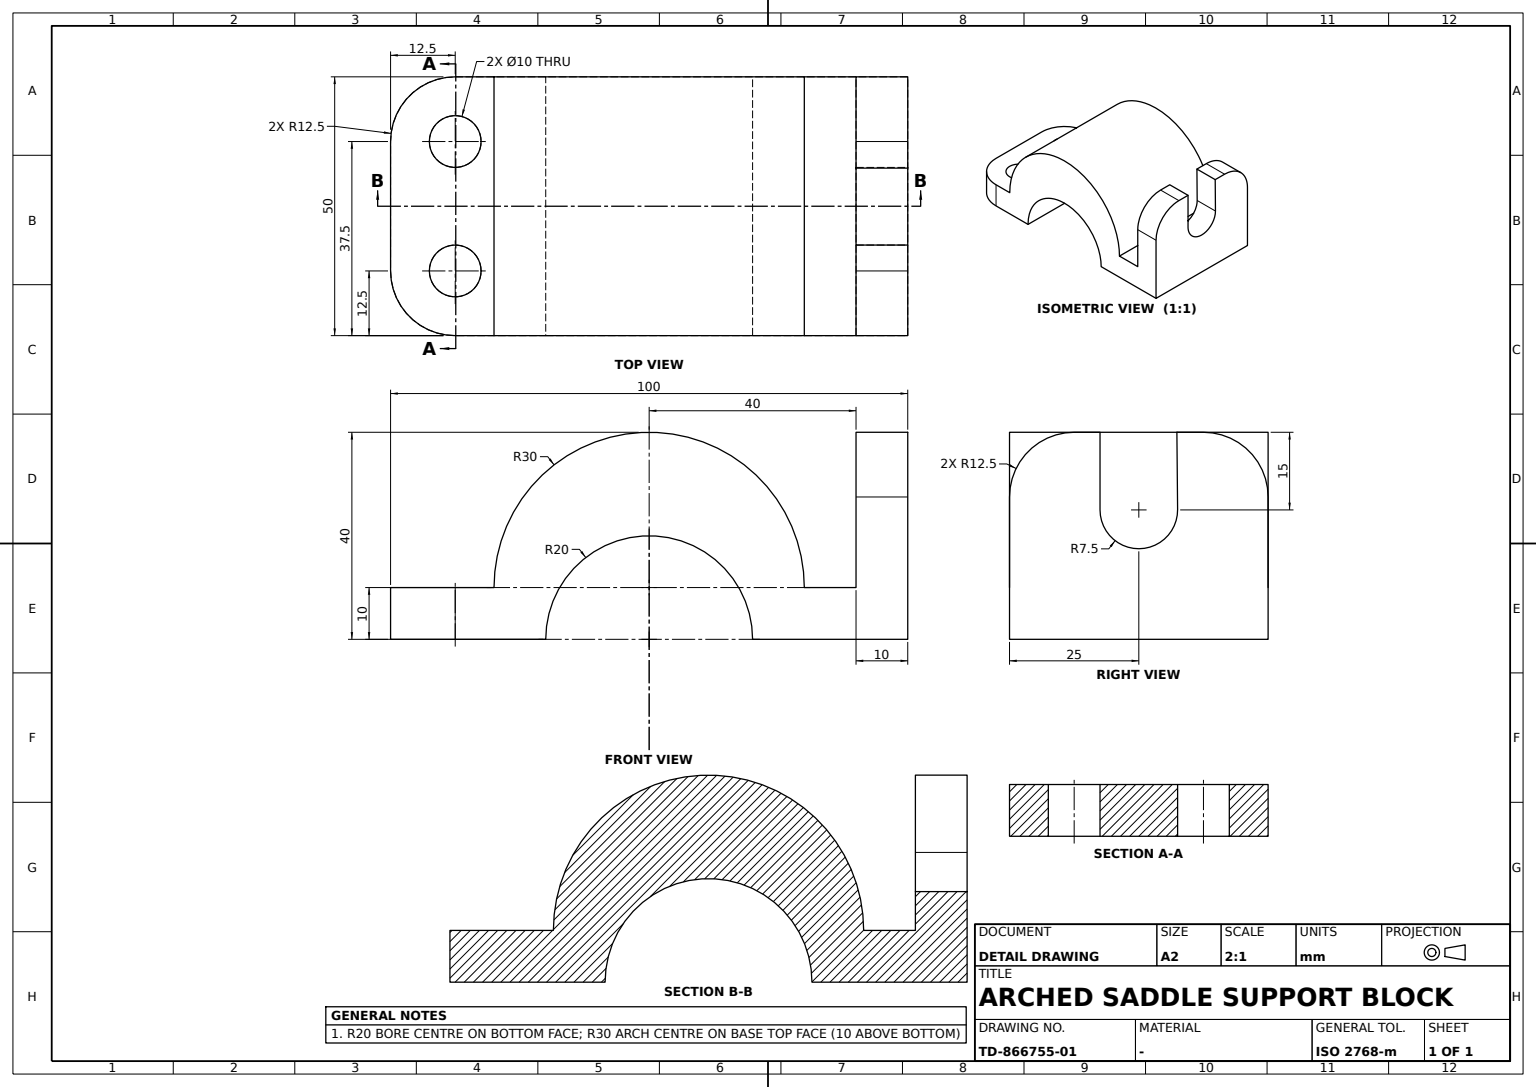
ISO-10303-21;
HEADER;
FILE_DESCRIPTION((''),'2;1');
FILE_NAME('','',(''),(''),'','','');
FILE_SCHEMA(('AUTOMOTIVE_DESIGN'));
ENDSEC;
DATA;
#1=APPLICATION_CONTEXT('');
#2=PRODUCT_CONTEXT('',#1,'mechanical');
#3=PRODUCT('','','',(#2));
#4=PRODUCT_DEFINITION_FORMATION('','',#3);
#5=PRODUCT_DEFINITION_CONTEXT('',#1,'design');
#6=PRODUCT_DEFINITION('','',#4,#5);
#7=PRODUCT_DEFINITION_SHAPE('','',#6);
#8=(LENGTH_UNIT()NAMED_UNIT(*)SI_UNIT(.MILLI.,.METRE.));
#9=(NAMED_UNIT(*)PLANE_ANGLE_UNIT()SI_UNIT($,.RADIAN.));
#10=(NAMED_UNIT(*)SI_UNIT($,.STERADIAN.)SOLID_ANGLE_UNIT());
#11=UNCERTAINTY_MEASURE_WITH_UNIT(LENGTH_MEASURE(0.005),#8,'distance_accuracy_value','');
#12=(GEOMETRIC_REPRESENTATION_CONTEXT(3)GLOBAL_UNCERTAINTY_ASSIGNED_CONTEXT((#11))GLOBAL_UNIT_ASSIGNED_CONTEXT((#8,#9,#10))REPRESENTATION_CONTEXT('',''));
#13=CARTESIAN_POINT('',(0.,-7.5,25.));
#14=VERTEX_POINT('',#13);
#15=CARTESIAN_POINT('',(-10.,-7.5,25.));
#16=VERTEX_POINT('',#15);
#17=CARTESIAN_POINT('',(-5.,-7.5,25.));
#18=DIRECTION('',(1.,0.,0.));
#19=VECTOR('',#18,1000.);
#20=LINE('',#17,#19);
#21=EDGE_CURVE('',#14,#16,#20,.F.);
#22=ORIENTED_EDGE('',*,*,#21,.T.);
#23=CARTESIAN_POINT('',(-10.,-7.5,40.));
#24=VERTEX_POINT('',#23);
#25=DIRECTION('',(0.,0.,1.));
#26=VECTOR('',#25,1000.);
#27=LINE('',#15,#26);
#28=EDGE_CURVE('',#16,#24,#27,.T.);
#29=ORIENTED_EDGE('',*,*,#28,.T.);
#30=CARTESIAN_POINT('',(0.,-7.5,40.));
#31=VERTEX_POINT('',#30);
#32=DIRECTION('',(-1.,0.,0.));
#33=VECTOR('',#32,1000.);
#34=LINE('',#30,#33);
#35=EDGE_CURVE('',#31,#24,#34,.T.);
#36=ORIENTED_EDGE('',*,*,#35,.F.);
#37=CARTESIAN_POINT('',(0.,-7.5,0.));
#38=LINE('',#37,#26);
#39=EDGE_CURVE('',#14,#31,#38,.T.);
#40=ORIENTED_EDGE('',*,*,#39,.F.);
#41=EDGE_LOOP('',(#22,#29,#36,#40));
#42=FACE_BOUND('',#41,.T.);
#43=DIRECTION('',(0.,-1.,0.));
#44=AXIS2_PLACEMENT_3D('',#13,#43,#25);
#45=PLANE('',#44);
#46=ADVANCED_FACE('',(#42),#45,.F.);
#47=CARTESIAN_POINT('',(-80.,-25.,10.));
#48=VERTEX_POINT('',#47);
#49=CARTESIAN_POINT('',(-20.,-25.,10.));
#50=VERTEX_POINT('',#49);
#51=CARTESIAN_POINT('',(-50.,-25.,10.));
#52=DIRECTION('',(0.,1.,0.));
#53=AXIS2_PLACEMENT_3D('',#51,#52,#25);
#54=CIRCLE('',#53,30.);
#55=EDGE_CURVE('',#48,#50,#54,.T.);
#56=ORIENTED_EDGE('',*,*,#55,.T.);
#57=CARTESIAN_POINT('',(-20.,25.,10.));
#58=VERTEX_POINT('',#57);
#59=VECTOR('',#52,1000.);
#60=LINE('',#49,#59);
#61=EDGE_CURVE('',#50,#58,#60,.T.);
#62=ORIENTED_EDGE('',*,*,#61,.T.);
#63=CARTESIAN_POINT('',(-80.,25.,10.));
#64=VERTEX_POINT('',#63);
#65=CARTESIAN_POINT('',(-50.,25.,10.));
#66=AXIS2_PLACEMENT_3D('',#65,#52,#25);
#67=CIRCLE('',#66,30.);
#68=EDGE_CURVE('',#64,#58,#67,.T.);
#69=ORIENTED_EDGE('',*,*,#68,.F.);
#70=LINE('',#47,#59);
#71=EDGE_CURVE('',#48,#64,#70,.T.);
#72=ORIENTED_EDGE('',*,*,#71,.F.);
#73=EDGE_LOOP('',(#56,#62,#69,#72));
#74=FACE_BOUND('',#73,.T.);
#75=CARTESIAN_POINT('',(-50.,0.,10.));
#76=AXIS2_PLACEMENT_3D('',#75,#52,#32);
#77=CYLINDRICAL_SURFACE('',#76,30.);
#78=ADVANCED_FACE('',(#74),#77,.T.);
#79=CARTESIAN_POINT('',(0.,7.362089,40.));
#80=VERTEX_POINT('',#79);
#81=CARTESIAN_POINT('',(0.,12.5,40.));
#82=VERTEX_POINT('',#81);
#83=CARTESIAN_POINT('',(0.,0.,40.));
#84=LINE('',#83,#59);
#85=EDGE_CURVE('',#80,#82,#84,.T.);
#86=ORIENTED_EDGE('',*,*,#85,.T.);
#87=CARTESIAN_POINT('',(-10.,12.5,40.));
#88=VERTEX_POINT('',#87);
#89=CARTESIAN_POINT('',(-50.,12.5,40.));
#90=LINE('',#89,#33);
#91=EDGE_CURVE('',#82,#88,#90,.T.);
#92=ORIENTED_EDGE('',*,*,#91,.T.);
#93=CARTESIAN_POINT('',(-10.,7.362089,40.));
#94=VERTEX_POINT('',#93);
#95=CARTESIAN_POINT('',(-10.,0.,40.));
#96=LINE('',#95,#59);
#97=EDGE_CURVE('',#94,#88,#96,.T.);
#98=ORIENTED_EDGE('',*,*,#97,.F.);
#99=LINE('',#79,#33);
#100=EDGE_CURVE('',#80,#94,#99,.T.);
#101=ORIENTED_EDGE('',*,*,#100,.F.);
#102=EDGE_LOOP('',(#86,#92,#98,#101));
#103=FACE_BOUND('',#102,.T.);
#104=DIRECTION('',(0.,0.,-1.));
#105=AXIS2_PLACEMENT_3D('',#83,#104,#32);
#106=PLANE('',#105);
#107=ADVANCED_FACE('',(#103),#106,.F.);
#108=CARTESIAN_POINT('',(-92.5,12.5,0.));
#109=VERTEX_POINT('',#108);
#110=CARTESIAN_POINT('',(-87.5,12.5,0.));
#111=AXIS2_PLACEMENT_3D('',#110,#104,#32);
#112=CIRCLE('',#111,5.);
#113=EDGE_CURVE('',#109,#109,#112,.T.);
#114=ORIENTED_EDGE('',*,*,#113,.T.);
#115=EDGE_LOOP('',(#114));
#116=FACE_BOUND('',#115,.T.);
#117=CARTESIAN_POINT('',(-82.5,12.5,10.));
#118=VERTEX_POINT('',#117);
#119=CARTESIAN_POINT('',(-87.5,12.5,10.));
#120=AXIS2_PLACEMENT_3D('',#119,#25,#18);
#121=CIRCLE('',#120,5.);
#122=EDGE_CURVE('',#118,#118,#121,.T.);
#123=ORIENTED_EDGE('',*,*,#122,.T.);
#124=EDGE_LOOP('',(#123));
#125=FACE_BOUND('',#124,.T.);
#126=CARTESIAN_POINT('',(-87.5,12.5,9.9));
#127=AXIS2_PLACEMENT_3D('',#126,#104,#18);
#128=CYLINDRICAL_SURFACE('',#127,5.);
#129=ADVANCED_FACE('',(#116,#125),#128,.F.);
#130=CARTESIAN_POINT('',(-10.,-12.5,40.));
#131=VERTEX_POINT('',#130);
#132=CARTESIAN_POINT('',(-10.,-25.,27.5));
#133=VERTEX_POINT('',#132);
#134=CARTESIAN_POINT('',(-10.,-12.5,27.5));
#135=AXIS2_PLACEMENT_3D('',#134,#18,#104);
#136=CIRCLE('',#135,12.5);
#137=EDGE_CURVE('',#131,#133,#136,.T.);
#138=ORIENTED_EDGE('',*,*,#137,.T.);
#139=CARTESIAN_POINT('',(0.,-25.,27.5));
#140=VERTEX_POINT('',#139);
#141=CARTESIAN_POINT('',(-50.,-25.,27.5));
#142=LINE('',#141,#33);
#143=EDGE_CURVE('',#140,#133,#142,.T.);
#144=ORIENTED_EDGE('',*,*,#143,.F.);
#145=CARTESIAN_POINT('',(0.,-12.5,40.));
#146=VERTEX_POINT('',#145);
#147=CARTESIAN_POINT('',(0.,-12.5,27.5));
#148=AXIS2_PLACEMENT_3D('',#147,#32,#25);
#149=CIRCLE('',#148,12.5);
#150=EDGE_CURVE('',#140,#146,#149,.T.);
#151=ORIENTED_EDGE('',*,*,#150,.T.);
#152=CARTESIAN_POINT('',(-50.,-12.5,40.));
#153=LINE('',#152,#33);
#154=EDGE_CURVE('',#146,#131,#153,.T.);
#155=ORIENTED_EDGE('',*,*,#154,.T.);
#156=EDGE_LOOP('',(#138,#144,#151,#155));
#157=FACE_BOUND('',#156,.T.);
#158=CARTESIAN_POINT('',(-50.,-12.5,27.5));
#159=AXIS2_PLACEMENT_3D('',#158,#32,#43);
#160=CYLINDRICAL_SURFACE('',#159,12.5);
#161=ADVANCED_FACE('',(#157),#160,.T.);
#162=CARTESIAN_POINT('',(-100.,12.5,0.));
#163=VERTEX_POINT('',#162);
#164=CARTESIAN_POINT('',(-100.,12.5,10.));
#165=VERTEX_POINT('',#164);
#166=CARTESIAN_POINT('',(-100.,12.5,20.));
#167=LINE('',#166,#26);
#168=EDGE_CURVE('',#163,#165,#167,.T.);
#169=ORIENTED_EDGE('',*,*,#168,.T.);
#170=CARTESIAN_POINT('',(-87.5,25.,10.));
#171=VERTEX_POINT('',#170);
#172=CIRCLE('',#120,12.5);
#173=EDGE_CURVE('',#171,#165,#172,.T.);
#174=ORIENTED_EDGE('',*,*,#173,.F.);
#175=CARTESIAN_POINT('',(-87.5,25.,0.));
#176=VERTEX_POINT('',#175);
#177=CARTESIAN_POINT('',(-87.5,25.,20.));
#178=LINE('',#177,#26);
#179=EDGE_CURVE('',#176,#171,#178,.T.);
#180=ORIENTED_EDGE('',*,*,#179,.F.);
#181=CIRCLE('',#111,12.5);
#182=EDGE_CURVE('',#163,#176,#181,.T.);
#183=ORIENTED_EDGE('',*,*,#182,.F.);
#184=EDGE_LOOP('',(#169,#174,#180,#183));
#185=FACE_BOUND('',#184,.T.);
#186=CARTESIAN_POINT('',(-87.5,12.5,20.));
#187=AXIS2_PLACEMENT_3D('',#186,#25,#32);
#188=CYLINDRICAL_SURFACE('',#187,12.5);
#189=ADVANCED_FACE('',(#185),#188,.T.);
#190=CARTESIAN_POINT('',(0.,-25.,0.));
#191=VERTEX_POINT('',#190);
#192=LINE('',#190,#26);
#193=EDGE_CURVE('',#191,#140,#192,.T.);
#194=ORIENTED_EDGE('',*,*,#193,.F.);
#195=CARTESIAN_POINT('',(0.,25.,0.));
#196=VERTEX_POINT('',#195);
#197=CARTESIAN_POINT('',(0.,0.,0.));
#198=LINE('',#197,#59);
#199=EDGE_CURVE('',#191,#196,#198,.T.);
#200=ORIENTED_EDGE('',*,*,#199,.T.);
#201=CARTESIAN_POINT('',(0.,25.,27.5));
#202=VERTEX_POINT('',#201);
#203=LINE('',#195,#26);
#204=EDGE_CURVE('',#196,#202,#203,.T.);
#205=ORIENTED_EDGE('',*,*,#204,.T.);
#206=CARTESIAN_POINT('',(0.,12.5,27.5));
#207=AXIS2_PLACEMENT_3D('',#206,#32,#25);
#208=CIRCLE('',#207,12.5);
#209=EDGE_CURVE('',#82,#202,#208,.T.);
#210=ORIENTED_EDGE('',*,*,#209,.F.);
#211=ORIENTED_EDGE('',*,*,#85,.F.);
#212=CARTESIAN_POINT('',(0.,7.499682,25.069112));
#213=VERTEX_POINT('',#212);
#214=CARTESIAN_POINT('',(0.,7.730045,0.071235));
#215=DIRECTION('',(0.,0.009214936,-0.999957542));
#216=VECTOR('',#215,1000.);
#217=LINE('',#214,#216);
#218=EDGE_CURVE('',#80,#213,#217,.T.);
#219=ORIENTED_EDGE('',*,*,#218,.T.);
#220=CARTESIAN_POINT('',(0.,0.,25.));
#221=AXIS2_PLACEMENT_3D('',#220,#32,#25);
#222=CIRCLE('',#221,7.5);
#223=EDGE_CURVE('',#14,#213,#222,.F.);
#224=ORIENTED_EDGE('',*,*,#223,.F.);
#225=ORIENTED_EDGE('',*,*,#39,.T.);
#226=EDGE_CURVE('',#146,#31,#84,.T.);
#227=ORIENTED_EDGE('',*,*,#226,.F.);
#228=ORIENTED_EDGE('',*,*,#150,.F.);
#229=EDGE_LOOP('',(#194,#200,#205,#210,#211,#219,#224,#225,#227,#228));
#230=FACE_BOUND('',#229,.T.);
#231=AXIS2_PLACEMENT_3D('',#197,#32,#25);
#232=PLANE('',#231);
#233=ADVANCED_FACE('',(#230),#232,.F.);
#234=CARTESIAN_POINT('',(-87.5,-25.,0.));
#235=VERTEX_POINT('',#234);
#236=CARTESIAN_POINT('',(-100.,-12.5,0.));
#237=VERTEX_POINT('',#236);
#238=CARTESIAN_POINT('',(-87.5,-12.5,0.));
#239=AXIS2_PLACEMENT_3D('',#238,#104,#32);
#240=CIRCLE('',#239,12.5);
#241=EDGE_CURVE('',#235,#237,#240,.T.);
#242=ORIENTED_EDGE('',*,*,#241,.F.);
#243=CARTESIAN_POINT('',(-87.5,-25.,10.));
#244=VERTEX_POINT('',#243);
#245=CARTESIAN_POINT('',(-87.5,-25.,20.));
#246=LINE('',#245,#26);
#247=EDGE_CURVE('',#235,#244,#246,.T.);
#248=ORIENTED_EDGE('',*,*,#247,.T.);
#249=CARTESIAN_POINT('',(-100.,-12.5,10.));
#250=VERTEX_POINT('',#249);
#251=CARTESIAN_POINT('',(-87.5,-12.5,10.));
#252=AXIS2_PLACEMENT_3D('',#251,#25,#18);
#253=CIRCLE('',#252,12.5);
#254=EDGE_CURVE('',#250,#244,#253,.T.);
#255=ORIENTED_EDGE('',*,*,#254,.F.);
#256=CARTESIAN_POINT('',(-100.,-12.5,20.));
#257=LINE('',#256,#26);
#258=EDGE_CURVE('',#237,#250,#257,.T.);
#259=ORIENTED_EDGE('',*,*,#258,.F.);
#260=EDGE_LOOP('',(#242,#248,#255,#259));
#261=FACE_BOUND('',#260,.T.);
#262=CARTESIAN_POINT('',(-87.5,-12.5,20.));
#263=AXIS2_PLACEMENT_3D('',#262,#25,#43);
#264=CYLINDRICAL_SURFACE('',#263,12.5);
#265=ADVANCED_FACE('',(#261),#264,.T.);
#266=ORIENTED_EDGE('',*,*,#179,.T.);
#267=CARTESIAN_POINT('',(0.,25.,10.));
#268=LINE('',#267,#19);
#269=EDGE_CURVE('',#171,#64,#268,.T.);
#270=ORIENTED_EDGE('',*,*,#269,.T.);
#271=ORIENTED_EDGE('',*,*,#68,.T.);
#272=CARTESIAN_POINT('',(-10.,25.,10.));
#273=VERTEX_POINT('',#272);
#274=CARTESIAN_POINT('',(-100.,25.,10.));
#275=LINE('',#274,#33);
#276=EDGE_CURVE('',#273,#58,#275,.T.);
#277=ORIENTED_EDGE('',*,*,#276,.F.);
#278=CARTESIAN_POINT('',(-10.,25.,27.5));
#279=VERTEX_POINT('',#278);
#280=CARTESIAN_POINT('',(-10.,25.,0.));
#281=VECTOR('',#104,1000.);
#282=LINE('',#280,#281);
#283=EDGE_CURVE('',#279,#273,#282,.T.);
#284=ORIENTED_EDGE('',*,*,#283,.F.);
#285=CARTESIAN_POINT('',(-50.,25.,27.5));
#286=LINE('',#285,#33);
#287=EDGE_CURVE('',#202,#279,#286,.T.);
#288=ORIENTED_EDGE('',*,*,#287,.F.);
#289=ORIENTED_EDGE('',*,*,#204,.F.);
#290=CARTESIAN_POINT('',(-30.,25.,0.));
#291=VERTEX_POINT('',#290);
#292=LINE('',#195,#33);
#293=EDGE_CURVE('',#196,#291,#292,.T.);
#294=ORIENTED_EDGE('',*,*,#293,.T.);
#295=CARTESIAN_POINT('',(-70.,25.,0.));
#296=VERTEX_POINT('',#295);
#297=CARTESIAN_POINT('',(-50.,25.,0.));
#298=AXIS2_PLACEMENT_3D('',#297,#52,#25);
#299=CIRCLE('',#298,20.);
#300=EDGE_CURVE('',#296,#291,#299,.T.);
#301=ORIENTED_EDGE('',*,*,#300,.F.);
#302=EDGE_CURVE('',#296,#176,#292,.T.);
#303=ORIENTED_EDGE('',*,*,#302,.T.);
#304=EDGE_LOOP('',(#266,#270,#271,#277,#284,#288,#289,#294,#301,#303));
#305=FACE_BOUND('',#304,.T.);
#306=AXIS2_PLACEMENT_3D('',#195,#52,#32);
#307=PLANE('',#306);
#308=ADVANCED_FACE('',(#305),#307,.T.);
#309=CARTESIAN_POINT('',(-30.,-25.,0.));
#310=VERTEX_POINT('',#309);
#311=LINE('',#309,#59);
#312=EDGE_CURVE('',#310,#291,#311,.T.);
#313=ORIENTED_EDGE('',*,*,#312,.T.);
#314=ORIENTED_EDGE('',*,*,#293,.F.);
#315=ORIENTED_EDGE('',*,*,#199,.F.);
#316=LINE('',#190,#33);
#317=EDGE_CURVE('',#191,#310,#316,.T.);
#318=ORIENTED_EDGE('',*,*,#317,.T.);
#319=EDGE_LOOP('',(#313,#314,#315,#318));
#320=FACE_BOUND('',#319,.T.);
#321=AXIS2_PLACEMENT_3D('',#197,#104,#32);
#322=PLANE('',#321);
#323=ADVANCED_FACE('',(#320),#322,.T.);
#324=ORIENTED_EDGE('',*,*,#61,.F.);
#325=CARTESIAN_POINT('',(-10.,-25.,10.));
#326=VERTEX_POINT('',#325);
#327=CARTESIAN_POINT('',(-100.,-25.,10.));
#328=LINE('',#327,#33);
#329=EDGE_CURVE('',#326,#50,#328,.T.);
#330=ORIENTED_EDGE('',*,*,#329,.F.);
#331=CARTESIAN_POINT('',(-10.,0.,10.));
#332=LINE('',#331,#59);
#333=EDGE_CURVE('',#326,#273,#332,.T.);
#334=ORIENTED_EDGE('',*,*,#333,.T.);
#335=ORIENTED_EDGE('',*,*,#276,.T.);
#336=EDGE_LOOP('',(#324,#330,#334,#335));
#337=FACE_BOUND('',#336,.T.);
#338=CARTESIAN_POINT('',(-100.,0.,10.));
#339=AXIS2_PLACEMENT_3D('',#338,#25,#18);
#340=PLANE('',#339);
#341=ADVANCED_FACE('',(#337),#340,.T.);
#342=ORIENTED_EDGE('',*,*,#113,.F.);
#343=EDGE_LOOP('',(#342));
#344=FACE_BOUND('',#343,.T.);
#345=CARTESIAN_POINT('',(-92.5,-12.5,0.));
#346=VERTEX_POINT('',#345);
#347=CIRCLE('',#239,5.);
#348=EDGE_CURVE('',#346,#346,#347,.T.);
#349=ORIENTED_EDGE('',*,*,#348,.F.);
#350=EDGE_LOOP('',(#349));
#351=FACE_BOUND('',#350,.T.);
#352=ORIENTED_EDGE('',*,*,#182,.T.);
#353=ORIENTED_EDGE('',*,*,#302,.F.);
#354=CARTESIAN_POINT('',(-70.,-25.,0.));
#355=VERTEX_POINT('',#354);
#356=LINE('',#354,#59);
#357=EDGE_CURVE('',#355,#296,#356,.T.);
#358=ORIENTED_EDGE('',*,*,#357,.F.);
#359=EDGE_CURVE('',#355,#235,#316,.T.);
#360=ORIENTED_EDGE('',*,*,#359,.T.);
#361=ORIENTED_EDGE('',*,*,#241,.T.);
#362=CARTESIAN_POINT('',(-100.,0.,0.));
#363=LINE('',#362,#59);
#364=EDGE_CURVE('',#237,#163,#363,.T.);
#365=ORIENTED_EDGE('',*,*,#364,.T.);
#366=EDGE_LOOP('',(#352,#353,#358,#360,#361,#365));
#367=FACE_BOUND('',#366,.T.);
#368=ADVANCED_FACE('',(#344,#351,#367),#322,.T.);
#369=ORIENTED_EDGE('',*,*,#35,.T.);
#370=EDGE_CURVE('',#131,#24,#96,.T.);
#371=ORIENTED_EDGE('',*,*,#370,.F.);
#372=ORIENTED_EDGE('',*,*,#154,.F.);
#373=ORIENTED_EDGE('',*,*,#226,.T.);
#374=EDGE_LOOP('',(#369,#371,#372,#373));
#375=FACE_BOUND('',#374,.T.);
#376=ADVANCED_FACE('',(#375),#106,.F.);
#377=CARTESIAN_POINT('',(-10.,-25.,0.));
#378=LINE('',#377,#281);
#379=EDGE_CURVE('',#133,#326,#378,.T.);
#380=ORIENTED_EDGE('',*,*,#379,.F.);
#381=ORIENTED_EDGE('',*,*,#137,.F.);
#382=ORIENTED_EDGE('',*,*,#370,.T.);
#383=ORIENTED_EDGE('',*,*,#28,.F.);
#384=CARTESIAN_POINT('',(-10.,7.499682,25.069112));
#385=VERTEX_POINT('',#384);
#386=CARTESIAN_POINT('',(-10.,0.,25.));
#387=AXIS2_PLACEMENT_3D('',#386,#18,#104);
#388=CIRCLE('',#387,7.5);
#389=EDGE_CURVE('',#16,#385,#388,.T.);
#390=ORIENTED_EDGE('',*,*,#389,.T.);
#391=CARTESIAN_POINT('',(-10.,7.357705,40.475719));
#392=LINE('',#391,#216);
#393=EDGE_CURVE('',#94,#385,#392,.T.);
#394=ORIENTED_EDGE('',*,*,#393,.F.);
#395=ORIENTED_EDGE('',*,*,#97,.T.);
#396=CARTESIAN_POINT('',(-10.,12.5,27.5));
#397=AXIS2_PLACEMENT_3D('',#396,#18,#104);
#398=CIRCLE('',#397,12.5);
#399=EDGE_CURVE('',#279,#88,#398,.T.);
#400=ORIENTED_EDGE('',*,*,#399,.F.);
#401=ORIENTED_EDGE('',*,*,#283,.T.);
#402=ORIENTED_EDGE('',*,*,#333,.F.);
#403=EDGE_LOOP('',(#380,#381,#382,#383,#390,#394,#395,#400,#401,#402));
#404=FACE_BOUND('',#403,.T.);
#405=AXIS2_PLACEMENT_3D('',#95,#18,#104);
#406=PLANE('',#405);
#407=ADVANCED_FACE('',(#404),#406,.F.);
#408=CARTESIAN_POINT('',(-5.,7.499682,25.069112));
#409=LINE('',#408,#19);
#410=EDGE_CURVE('',#213,#385,#409,.F.);
#411=ORIENTED_EDGE('',*,*,#410,.F.);
#412=ORIENTED_EDGE('',*,*,#218,.F.);
#413=ORIENTED_EDGE('',*,*,#100,.T.);
#414=ORIENTED_EDGE('',*,*,#393,.T.);
#415=EDGE_LOOP('',(#411,#412,#413,#414));
#416=FACE_BOUND('',#415,.T.);
#417=CARTESIAN_POINT('',(0.,7.357705,40.475719));
#418=DIRECTION('',(0.,0.999957542,0.009214936));
#419=AXIS2_PLACEMENT_3D('',#417,#418,#215);
#420=PLANE('',#419);
#421=ADVANCED_FACE('',(#416),#420,.F.);
#422=ORIENTED_EDGE('',*,*,#287,.T.);
#423=ORIENTED_EDGE('',*,*,#399,.T.);
#424=ORIENTED_EDGE('',*,*,#91,.F.);
#425=ORIENTED_EDGE('',*,*,#209,.T.);
#426=EDGE_LOOP('',(#422,#423,#424,#425));
#427=FACE_BOUND('',#426,.T.);
#428=CARTESIAN_POINT('',(-50.,12.5,27.5));
#429=AXIS2_PLACEMENT_3D('',#428,#32,#25);
#430=CYLINDRICAL_SURFACE('',#429,12.5);
#431=ADVANCED_FACE('',(#427),#430,.T.);
#432=CARTESIAN_POINT('',(-82.5,-12.5,10.));
#433=VERTEX_POINT('',#432);
#434=CIRCLE('',#252,5.);
#435=EDGE_CURVE('',#433,#433,#434,.T.);
#436=ORIENTED_EDGE('',*,*,#435,.T.);
#437=EDGE_LOOP('',(#436));
#438=FACE_BOUND('',#437,.T.);
#439=ORIENTED_EDGE('',*,*,#348,.T.);
#440=EDGE_LOOP('',(#439));
#441=FACE_BOUND('',#440,.T.);
#442=CARTESIAN_POINT('',(-87.5,-12.5,9.9));
#443=AXIS2_PLACEMENT_3D('',#442,#104,#18);
#444=CYLINDRICAL_SURFACE('',#443,5.);
#445=ADVANCED_FACE('',(#438,#441),#444,.F.);
#446=ORIENTED_EDGE('',*,*,#55,.F.);
#447=CARTESIAN_POINT('',(0.,-25.,10.));
#448=LINE('',#447,#19);
#449=EDGE_CURVE('',#244,#48,#448,.T.);
#450=ORIENTED_EDGE('',*,*,#449,.F.);
#451=ORIENTED_EDGE('',*,*,#247,.F.);
#452=ORIENTED_EDGE('',*,*,#359,.F.);
#453=CARTESIAN_POINT('',(-50.,-25.,0.));
#454=AXIS2_PLACEMENT_3D('',#453,#52,#25);
#455=CIRCLE('',#454,20.);
#456=EDGE_CURVE('',#355,#310,#455,.T.);
#457=ORIENTED_EDGE('',*,*,#456,.T.);
#458=ORIENTED_EDGE('',*,*,#317,.F.);
#459=ORIENTED_EDGE('',*,*,#193,.T.);
#460=ORIENTED_EDGE('',*,*,#143,.T.);
#461=ORIENTED_EDGE('',*,*,#379,.T.);
#462=ORIENTED_EDGE('',*,*,#329,.T.);
#463=EDGE_LOOP('',(#446,#450,#451,#452,#457,#458,#459,#460,#461,#462));
#464=FACE_BOUND('',#463,.T.);
#465=AXIS2_PLACEMENT_3D('',#190,#52,#32);
#466=PLANE('',#465);
#467=ADVANCED_FACE('',(#464),#466,.F.);
#468=ORIENTED_EDGE('',*,*,#389,.F.);
#469=ORIENTED_EDGE('',*,*,#21,.F.);
#470=ORIENTED_EDGE('',*,*,#223,.T.);
#471=ORIENTED_EDGE('',*,*,#410,.T.);
#472=EDGE_LOOP('',(#468,#469,#470,#471));
#473=FACE_BOUND('',#472,.T.);
#474=CARTESIAN_POINT('',(-5.,0.,25.));
#475=AXIS2_PLACEMENT_3D('',#474,#18,#52);
#476=CYLINDRICAL_SURFACE('',#475,7.5);
#477=ADVANCED_FACE('',(#473),#476,.F.);
#478=ORIENTED_EDGE('',*,*,#456,.F.);
#479=ORIENTED_EDGE('',*,*,#357,.T.);
#480=ORIENTED_EDGE('',*,*,#300,.T.);
#481=ORIENTED_EDGE('',*,*,#312,.F.);
#482=EDGE_LOOP('',(#478,#479,#480,#481));
#483=FACE_BOUND('',#482,.T.);
#484=CARTESIAN_POINT('',(-50.,0.,0.));
#485=AXIS2_PLACEMENT_3D('',#484,#52,#32);
#486=CYLINDRICAL_SURFACE('',#485,20.);
#487=ADVANCED_FACE('',(#483),#486,.F.);
#488=ORIENTED_EDGE('',*,*,#71,.T.);
#489=ORIENTED_EDGE('',*,*,#269,.F.);
#490=ORIENTED_EDGE('',*,*,#173,.T.);
#491=LINE('',#338,#59);
#492=EDGE_CURVE('',#250,#165,#491,.T.);
#493=ORIENTED_EDGE('',*,*,#492,.F.);
#494=ORIENTED_EDGE('',*,*,#254,.T.);
#495=ORIENTED_EDGE('',*,*,#449,.T.);
#496=EDGE_LOOP('',(#488,#489,#490,#493,#494,#495));
#497=FACE_BOUND('',#496,.T.);
#498=ORIENTED_EDGE('',*,*,#435,.F.);
#499=EDGE_LOOP('',(#498));
#500=FACE_BOUND('',#499,.T.);
#501=ORIENTED_EDGE('',*,*,#122,.F.);
#502=EDGE_LOOP('',(#501));
#503=FACE_BOUND('',#502,.T.);
#504=ADVANCED_FACE('',(#497,#500,#503),#340,.T.);
#505=ORIENTED_EDGE('',*,*,#258,.T.);
#506=ORIENTED_EDGE('',*,*,#492,.T.);
#507=ORIENTED_EDGE('',*,*,#168,.F.);
#508=ORIENTED_EDGE('',*,*,#364,.F.);
#509=EDGE_LOOP('',(#505,#506,#507,#508));
#510=FACE_BOUND('',#509,.T.);
#511=AXIS2_PLACEMENT_3D('',#362,#32,#25);
#512=PLANE('',#511);
#513=ADVANCED_FACE('',(#510),#512,.T.);
#514=CLOSED_SHELL('',(#46,#78,#107,#129,#161,#189,#233,#265,#308,#323,#341,#368,#376,#407,#421,#431,#445,#467,#477,#487,#504,#513));
#515=MANIFOLD_SOLID_BREP('',#514);
#516=ADVANCED_BREP_SHAPE_REPRESENTATION('',(#515),#12);
#517=SHAPE_DEFINITION_REPRESENTATION(#7,#516);
ENDSEC;
END-ISO-10303-21;
